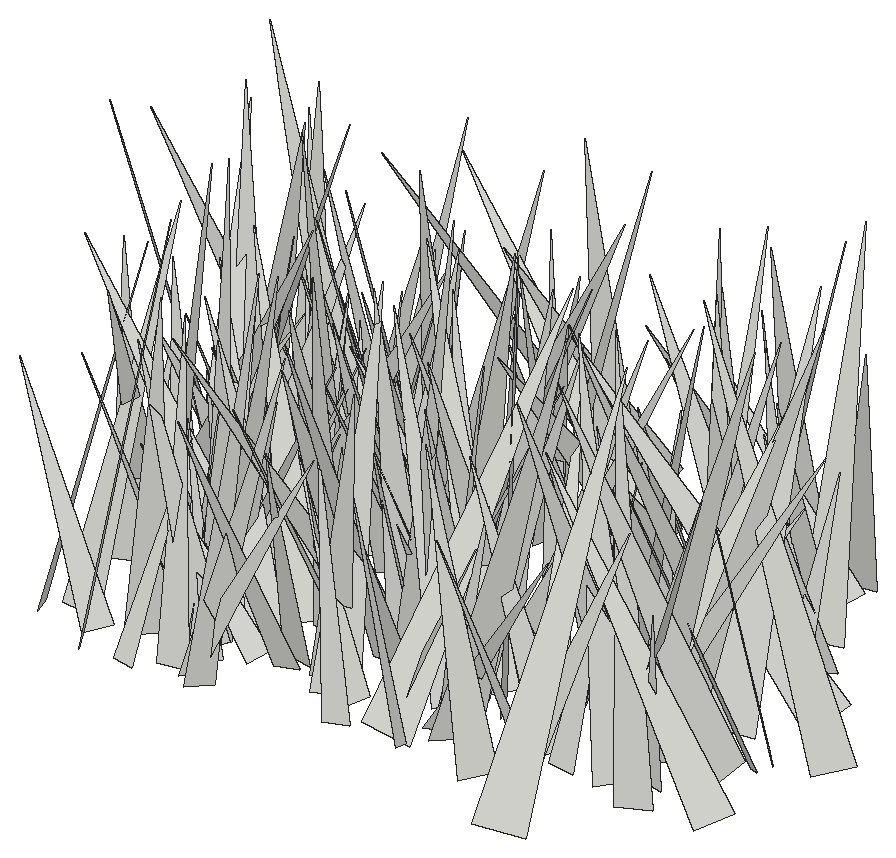
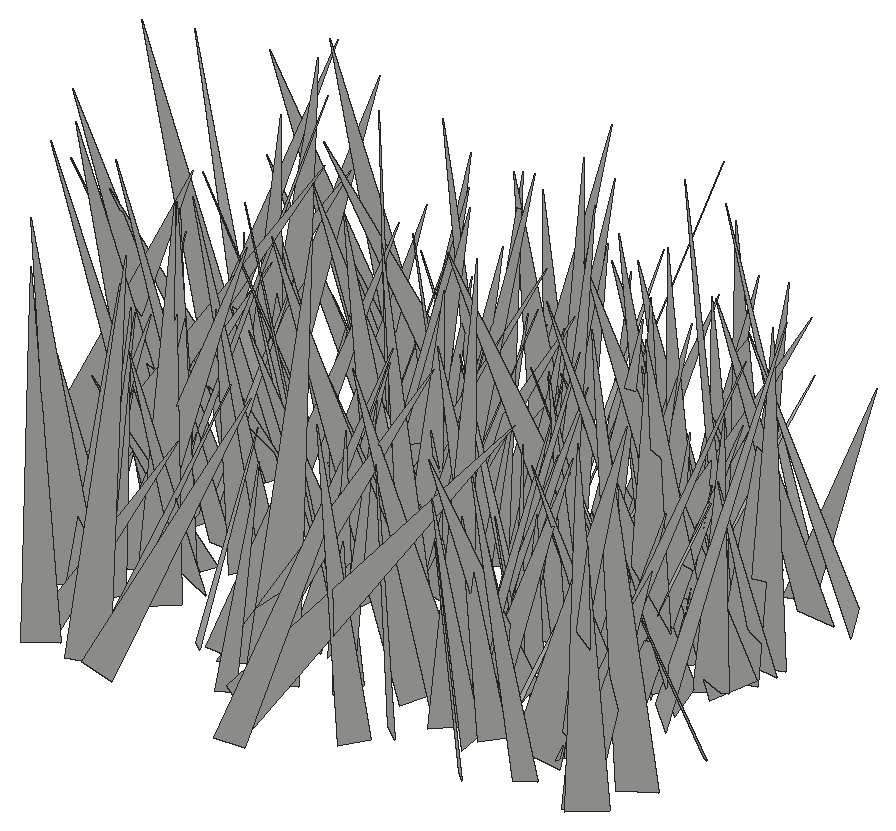
# SketchUp Ruby script. Lengths in inches.
U = 1.inch
M = Sketchup.active_model
def pt(a) = Geom::Point3d.new(a.map { |v| v * U })
def face(e, loops, mat)
  f = e.add_face(loops[0].map { |a| pt(a) })
  loops[1..].each { |l| e.add_face(l.map { |a| pt(a) }).erase! }
  f.material = f.back_material = mat if mat
  f
end
# faces: each face lists its corners as indices into pts; further lists are holes
def faces(e, pts, list, mat = nil) = list.each { |f| face(e, (f[0].is_a?(Array) ? f : [f]).map { |l| l.map { |i| pts[i] } }, mat) }
# xy, xz, yz: faces in a plane at the given z, y or x. An outline is a flat list of corners, or four numbers for a rectangle; further outlines are holes
def ring(l) = l.size == 4 ? [[l[0], l[1]], [l[2], l[1]], [l[2], l[3]], [l[0], l[3]]] : l.each_slice(2).to_a
def flat(e, list, mat, &to3) = list.each { |f| face(e, (f[0].is_a?(Array) ? f : [f]).map { |l| ring(l).map { |u, v| to3.(u, v) } }, mat) }
def xy(e, z, list, mat = nil) = flat(e, list, mat) { |x, y| [x, y, z] }
def xz(e, y, list, mat = nil) = flat(e, list, mat) { |x, z| [x, y, z] }
def yz(e, x, list, mat = nil) = flat(e, list, mat) { |y, z| [x, y, z] }
def lines(e, pts, list) = list.each { |a, b| e.add_line(pt(pts[a]), pt(pts[b])) }
# prism: a flat outline (further loops are holes) pulled along v
def prism(e, loops, v, mat = nil)
  f = face(e, loops, mat); d = Geom::Vector3d.new(v.map { |x| x * U })
  f.pushpull(f.normal.samedirection?(d) ? d.length : -d.length)
end
def box(e, o, s, mat = nil) = prism(e, [[o, [o[0] + s[0], o[1], o[2]], [o[0] + s[0], o[1] + s[1], o[2]], [o[0], o[1] + s[1], o[2]]]], [0, 0, s[2]], mat)
def at(x, y, z, deg = 0) = Geom::Transformation.translation(pt([x, y, z])) * Geom::Transformation.rotation(ORIGIN, Z_AXIS, deg.degrees)
def axes(o, x, y, z) = Geom::Transformation.new([*x, 0, *y, 0, *z, 0, *pt(o).to_a, 1])
def part(name) = M.definitions.add(name)
# library, detail: a bought-in or finely detailed component or shape, given as its bounding box
def library(name, o, s) = part(name).tap { |d| box(d.entities, o, s) }
def detail(e, o, s) = box(e.add_group.entities, o, s)
def put(e, d, t, mat = nil) = e.add_instance(d, t).tap { |i| i.material = mat if mat }
def group(e, t, mat = nil) = e.add_group.tap { |g| g.transformation = t; g.material = mat if mat }.entities
root = M.entities
c1 = part("fur_instance\#9")
p = [[0.8125,0,1.79],[0.67,-0.02,1.48],[0,-0.11,0],[0,0.11,0]]
faces(c1.entities,p,[[0,1,2,3]])
put(root,c1,axes([129.59,252.91,-27.1],[-4.54367,3.48057,1.82928],[3.81076,4.58683,0.73803],[0.96889,-1.71821,5.67579]))
put(root,c1,axes([114.01,252.82,-27.1],[-3.48001,3.233,0.8636],[3.33945,3.27515,1.19585],[-0.21495,-1.45934,4.59703]))
put(root,c1,axes([117.92,252.73,-27.1],[2.74788,4.31889,0.7575],[4.17328,-2.30167,-2.01583],[1.34551,-1.68135,4.70533]))
put(root,c1,axes([116.02,251.58,-27.1],[0.74131,3.87524,0.12897],[3.87698,-0.74271,0.03187],[-0.05555,-0.12068,3.94537]))
put(root,c1,axes([115.4,253.56,-27.1],[-4.12278,4.06528,3.37823],[4.64279,4.83304,-0.14992],[2.52655,-2.24755,5.78803]))
put(root,c1,axes([120.35,254.6,-27.1],[-0.32554,-5.06602,0.7464],[-4.99056,0.14633,-1.18345],[-1.14716,0.80105,4.9366]))
put(root,c1,axes([132.36,250.52,-27.1],[-3.86216,7.0455,1.20437],[6.7899,4.04407,-1.88376],[2.2331,-0.11104,7.81068]))
put(root,c1,axes([123.87,252.73,-27.1],[-0.78367,4.54033,1.31363],[4.69244,0.5877,0.76808],[-0.56674,-1.41222,4.54299]))
put(root,c1,axes([113.97,252.05,-27.1],[6.26441,4.08516,1.86388],[4.05019,-6.52197,0.68206],[-1.9387,-0.42509,7.44756]))
put(root,c1,axes([117.64,254.12,-27.1],[-4.95355,2.49117,1.9463],[2.93301,4.97148,1.10159],[1.17959,-1.90003,5.43416]))
put(root,c1,axes([130.23,254.6,-27.1],[-3.91317,-2.34388,0.53173],[-2.28614,3.94348,0.55853],[0.74167,-0.21123,4.52711]))
put(root,c1,axes([117.44,252.4,-27.1],[-0.20928,5.81187,1.2771],[5.90875,0.05179,0.73257],[-0.70395,-1.2931,5.76932]))
put(root,c1,axes([118.37,252.4,-27.1],[5.34451,-1.51745,2.02584],[-2.07356,-5.33917,1.4711],[-1.45157,2.03988,5.35746]))
put(root,c1,axes([131.07,252.87,-27.1],[0.51844,5.23573,1.343],[5.13497,-0.0558,-1.76472],[1.68777,-1.43851,4.95655]))
put(root,c1,axes([120.26,255.23,-27.1],[0.02895,-4.95019,0.58964],[-4.94989,0.0415,0.59139],[0.59214,0.58889,4.91483]))
put(root,c1,axes([126.4,252.91,-27.1],[-4.21104,-1.2398,0.43934],[-1.31531,3.95873,-1.43574],[-0.00925,1.50143,4.14832]))
put(root,c1,axes([125.05,254.18,-27.1],[3.85978,2.30102,0.3483],[2.28006,-3.60384,-1.45862],[0.46617,-1.42533,4.2503]))
put(root,c1,axes([117.06,254.07,-27.1],[-4.69197,-2.31538,0.05263],[-2.28134,4.60011,-1.00642],[-0.39908,0.92541,5.13447]))
put(root,c1,axes([121.87,254.95,-27.1],[3.13383,-5.16211,1.39491],[-5.34355,-3.08346,0.59403],[-0.19921,1.50298,6.00961]))
put(root,c1,axes([118.89,251.94,-27.1],[-6.51752,1.2418,2.00991],[0.54856,6.53189,-2.25684],[2.29801,1.9627,6.23913]))
put(root,c1,axes([119.2,254.6,-27.1],[-3.24563,2.42896,0.17461],[2.25293,2.88449,1.75171],[-0.92447,-1.49811,3.65588]))
put(root,c1,axes([122.88,256.92,-27.1],[-0.43608,-7.58063,0.50958],[-7.59761,0.43802,0.01424],[0.04352,0.50791,7.59315]))
put(root,c1,axes([118.24,253.43,-27.1],[-3.93894,0.78438,0.2139],[0.7314,3.88076,-0.76228],[0.35506,0.70765,3.94328]))
put(root,c1,axes([123.49,254.3,-27.1],[-4.0044,1.49429,0.5536],[1.5481,4.00291,0.3933],[0.37782,-0.56428,4.25599]))
put(root,c1,axes([122.49,255.03,-27.1],[-1.30736,-3.53096,1.01989],[-3.67333,1.2908,-0.2398],[0.12042,1.04076,3.75757]))
put(root,c1,axes([121.07,256.91,-27.1],[-3.83453,-4.44323,0.31037],[-4.29048,3.7947,1.3169],[1.19597,-0.63261,5.71941]))
put(root,c1,axes([126.65,254.46,-27.1],[3.7348,-2.45498,0.02516],[-2.33086,-3.53122,1.44009],[0.77113,1.21649,4.23106]))
put(root,c1,axes([117.09,253.32,-27.1],[2.12896,3.50938,0.78952],[3.35263,-2.26833,1.04217],[-1.30344,-0.10245,3.97015]))
put(root,c1,axes([127.47,254.32,-27.1],[7.2049,-3.47591,1.96261],[-3.83046,-7.15988,1.38131],[-1.1231,2.12096,7.87937]))
put(root,c1,axes([119.89,259.11,-27.1],[-6.50454,-4.83681,0.42708],[-4.2184,5.98256,3.50717],[2.40464,-2.5885,7.30777]))
put(root,c1,axes([111.64,252.9,-27.1],[5.51365,3.20537,1.24598],[2.89904,-5.59864,1.57419],[-1.84998,0.77981,6.18035]))
put(root,c1,axes([130.52,255.7,-27.1],[-4.35819,2.96505,1.59627],[3.3258,4.19926,1.28011],[0.52792,-1.97688,5.11338]))
put(root,c1,axes([133.25,257,-27.1],[1.43067,-7.01564,1.7352],[-6.90944,-1.84641,-1.76845],[-2.11892,1.28394,6.9382]))
put(root,c1,axes([137.39,255.32,-27.1],[-4.14935,5.21761,0.66717],[4.85978,3.47746,3.02911],[-2.01273,-2.35998,5.93844]))
put(root,c1,axes([120.62,258.33,-27.1],[5.40488,-4.57462,0.50738],[-4.27322,-5.27816,-2.06831],[-1.71004,-1.26929,6.77215]))
put(root,c1,axes([122.66,254.21,-27.1],[-3.77046,5.93467,2.17976],[6.06315,4.1134,-0.71146],[1.79161,-1.43096,6.99504]))
put(root,c1,axes([134.34,255.89,-27.1],[-0.14412,-3.47359,1.04669],[-3.58722,0.2928,0.47779],[0.54152,1.01518,3.44359]))
put(root,c1,axes([132.18,257.37,-27.1],[7.41722,0.99885,0.34739],[1.05742,-6.96886,-2.53978],[0.01548,-2.56338,7.04006]))
put(root,c1,axes([126.39,255.35,-27.1],[0.00091,-3.67707,1.93886],[-4.08733,0.35251,0.67045],[0.75747,1.90654,3.61543]))
put(root,c1,axes([112.81,253.43,-27.1],[0.72086,7.11073,0.81641],[7.15729,-0.71063,-0.13028],[0.04812,-0.82534,7.14599]))
put(root,c1,axes([133.4,255.4,-27.1],[-5.88987,4.84378,2.23578],[5.14185,6.04195,0.45575],[1.42207,-1.78441,7.61217]))
put(root,c1,axes([131.36,254.9375,-27.1],[0.22863,4.55848,1.01522],[4.65358,-0.13679,-0.43379],[0.39321,-1.03161,4.54355]))
put(root,c1,axes([135.82,257.82,-27.1],[-7.8024,0.71377,1.7229],[1.19599,7.6017,2.26696],[1.43089,-2.46171,7.49986]))
put(root,c1,axes([112.16,258.375,-27.1],[2.77965,-6.05851,0.20454],[-6.05263,-2.78627,-0.276],[-0.3362,0.0706,6.66001]))
put(root,c1,axes([118,256.51,-27.1],[-6.653,2.83628,0.09553],[2.75112,6.38619,1.99099],[-0.69638,-1.86767,6.95291]))
put(root,c1,axes([120.18,257.19,-27.1],[-0.4517,-7.27096,2.0225],[-7.50286,0.65147,0.6664],[0.81515,1.96726,7.25444]))
put(root,c1,axes([116.52,256.22,-27.1],[6.38697,-1.69717,1.73981],[-1.81592,-6.58358,0.24416],[-1.61547,0.69051,6.6041]))
put(root,c1,axes([125.53,253.21,-27.1],[-1.37451,8.097,0.63904],[7.82187,1.49419,-2.10823],[2.18815,-0.25501,7.93763]))
put(root,c1,axes([126.71,254.72,-27.1],[3.29752,4.92899,1.52703],[4.76096,-3.60504,1.35547],[-1.98997,-0.45731,5.77332]))
put(root,c1,axes([113.85,256.53,-27.1],[4.80804,6.17674,2.98381],[6.78482,-4.81897,-0.95722],[-1.01068,-2.96612,7.76873]))
put(root,c1,axes([134.84,254.35,-27.1],[-0.02832,7.80203,1.3013],[7.5934,-0.33756,2.1891],[-2.2148,-1.25708,7.48868]))
put(root,c1,axes([117.64,254.31,-27.1],[-7.86516,0.65945,1.92725],[0.13584,7.83978,-2.12819],[2.03241,2.02799,7.60042]))
put(root,c1,axes([116.55,256.39,-27.1],[3.89931,-1.45547,0.98195],[-1.58431,-3.9476,0.44006],[-0.75669,0.76505,4.13877]))
put(root,c1,axes([112.03,257.02,-27.1],[2.29625,-5.32789,2.30917],[-5.72704,-2.48806,-0.04565],[-0.95905,2.10109,5.80148]))
put(root,c1,axes([123.34,257.37,-27.1],[3.99451,-5.40043,2.70776],[-5.64329,-4.49426,-0.63847],[-2.15638,1.75774,6.68679]))
put(root,c1,axes([123.23,257.58,-27.1],[-1.72033,-4.15588,1.09836],[-4.2769,1.77348,0.01157],[0.4311,1.01028,4.49785]))
put(root,c1,axes([116.7,256.26,-27.1],[0.17252,3.92598,1.26935],[3.97591,-0.49782,0.99933],[-1.10305,-1.18034,3.80058]))
put(root,c1,axes([125.57,257.53,-27.1],[-2.41735,-5.08882,0.8159],[-4.81582,1.90935,-2.35956],[-1.83565,1.69223,5.11586]))
put(root,c1,axes([117.93,257.56,-27.1],[-5.02237,2.51021,1.68016],[2.86774,4.98644,1.12241],[0.94877,-1.78398,5.50142]))
put(root,c1,axes([125.96,256.1,-27.1],[-6.07575,2.79462,0.62219],[2.80321,6.10345,-0.04049],[0.58225,-0.22305,6.68752]))
put(root,c1,axes([123.87,256.27,-27.1],[3.41828,7.22194,2.57308],[7.56489,-3.63472,0.1519],[-1.24484,-2.25703,7.98861]))
put(root,c1,axes([115.95,256.41,-27.1],[-2.49427,4.27012,1.59064],[4.35584,2.76683,-0.59729],[1.33819,-1.04698,4.90903]))
put(root,c1,axes([118.85,255.46,-27.1],[-2.09774,5.99421,0.07606],[5.73274,1.98235,1.88224],[-1.75272,-0.69034,6.06533]))
put(root,c1,axes([116.13,256.1,-27.1],[4.9565,-0.0282,0.53243],[-0.1703,-4.80111,1.33099],[-0.50525,1.34155,4.77453]))
put(root,c1,axes([124.52,258.66,-27.1],[-3.87512,-3.17972,0.32504],[-3.163,3.88842,0.32938],[0.4601,-0.04943,5.00187]))
put(root,c1,axes([121.32,259.05,-27.1],[-2.38013,-2.88459,0.25848],[-2.75196,2.35686,0.96161],[0.90246,-0.42079,3.61403]))
put(root,c1,axes([125.82,259.48,-27.1],[3.87648,-5.20572,1.47803],[-5.00062,-4.14086,-1.46909],[-2.0683,0.2548,6.32205]))
put(root,c1,axes([127.39,256.97,-27.1],[6.18055,4.14964,3.19418],[4.26505,-6.85588,0.65402],[-3.03836,-1.18276,7.41558]))
put(root,c1,axes([125.02,258.51,-27.1],[-0.19276,-5.01478,1.27598],[-5.16585,0.1124,-0.33865],[-0.30027,1.28555,5.00705]))
put(root,c1,axes([118.4,259.92,-27.1],[4.15376,-5.21591,0.7578],[-5.12927,-4.22232,-0.94677],[-1.21268,-0.00681,6.60024]))
put(root,c1,axes([126.24,256.61,-27.1],[6.10707,-2.19869,2.10682],[-2.76305,-5.98564,1.76265],[-1.28003,2.43046,6.24689]))
put(root,c1,axes([123.23,260.01,-27.1],[-2.01035,-7.12989,1.00319],[-7.18316,2.0575,0.22838],[0.49393,0.90254,7.40437]))
put(root,c1,axes([132.33,257.89,-27.1],[6.94828,-4.27135,1.74082],[-4.55894,-6.83788,1.41876],[-0.70067,2.13364,8.03182]))
put(root,c1,axes([126.39,259.63,-27.1],[-6.42762,0.7775,0.36666],[0.8533,6.10569,2.01137],[0.10407,-2.04186,6.15412]))
put(root,c1,axes([118.98,257.37,-27.1],[-4.49285,4.90641,0.97236],[5.00159,4.41981,0.80831],[0.04935,-1.26349,6.60342]))
put(root,c1,axes([111.85,257.19,-27.1],[0.3484,4.1984,0.59349],[4.23915,-0.35779,0.04247],[-0.09183,-0.58788,4.21262]))
put(root,c1,axes([126.6,257.47,-27.1],[-5.45873,5.352,1.02249],[5.44819,5.38274,0.9113],[0.08123,-1.36725,7.5902]))
put(root,c1,axes([136.29,258.72,-27.1],[-3.48224,-3.77241,0.29956],[-3.58403,3.15695,-1.90663],[-1.21472,1.49981,4.76674]))
put(root,c1,axes([116.47,258.5625,-27.1],[3.59656,-0.31618,0.04156],[-0.31764,-3.59357,0.14939],[-0.02828,0.15246,3.60734]))
put(root,c1,axes([118.32,259.29,-27.1],[-3.2308,-2.41105,0.08917],[-2.40238,3.20101,-0.49122],[-0.22293,0.4467,4.00124]))
put(root,c1,axes([114.16,259.76,-27.1],[3.91302,0.34843,0.25725],[0.41449,-3.69091,-1.30566],[-0.12562,-1.32482,3.70519]))
put(root,c1,axes([111.92,258.78,-27.1],[6.68383,-3.60485,0.36068],[-3.59385,-6.50181,1.61538],[0.45749,1.59067,7.42019]))
put(root,c1,axes([130.04,258.8,-27.1],[-4.57594,-0.69447,0.70937],[-0.73517,4.61906,-0.2203],[0.6671,0.32667,4.62309]))
put(root,c1,axes([115.96,258.54,-27.1],[4.04604,3.23344,0.3968],[3.2461,-3.94826,-0.92578],[0.27467,-0.96906,5.09593]))
put(root,c1,axes([115.92,260.46,-27.1],[0.4513,-4.46287,0.47479],[-4.46772,-0.49211,-0.3789],[-0.42669,0.43236,4.4696]))
put(root,c1,axes([132.03,260.8,-27.1],[-2.1706,-3.79382,0.07549],[-3.76138,2.16267,0.53397],[0.50075,-0.20018,4.33814]))
put(root,c1,axes([113.86,259.62,-27.1],[2.36967,1.89121,2.13493],[2.35412,-2.86396,-0.07595],[-1.61018,-1.40392,3.03088]))
put(root,c1,axes([124.71,257.41,-27.1],[0.6459,3.9486,0.07217],[3.68247,-0.62859,1.43463],[-1.42692,0.16515,3.73504]))
put(root,c1,axes([136.28,259.63,-27.1],[-3.38614,-3.10021,1.02366],[-3.22386,3.40798,-0.34286],[0.51569,0.94841,4.57818]))
put(root,c1,axes([112.42,259.33,-27.1],[2.60909,-3.89298,2.22887],[-4.24925,-2.97119,-0.21539],[-1.4377,1.71676,4.68148]))
put(root,c1,axes([132.41,256.97,-27.1],[-1.13308,6.40977,0.66119],[6.08836,1.28481,-2.02171],[2.11049,-0.26515,6.18722]))
put(root,c1,axes([113.86,261.7,-27.1],[3.91388,-2.85851,1.41513],[-2.09693,-3.9939,-2.26798],[-2.40345,-1.17037,4.2832]))
put(root,c1,axes([118.05,258.32,-27.1],[0.83118,5.18677,1.07004],[5.28228,-0.88982,0.21009],[-0.38088,-1.02179,5.24874]))
put(root,c1,axes([129.16,259.1,-27.1],[-3.23487,-1.73884,2.61208],[-2.22596,3.91581,-0.14997],[2.2117,1.39779,3.66954]))
put(root,c1,axes([118.47,259.98,-27.1],[-2.90002,-7.26429,3.03178],[-7.85451,2.88308,-0.60516],[0.51793,3.0479,7.79832]))
put(root,c1,axes([115.9375,259.31,-27.1],[5.9864,-4.39629,0.74457],[-4.35138,-5.48795,2.58196],[0.97326,2.50473,6.96403]))
put(root,c1,axes([132.49,262.61,-27.1],[-7.22673,-3.69522,1.05519],[-3.3656,7.17065,2.06111],[1.85494,-1.38592,7.85061]))
put(root,c1,axes([122.51,259.36,-27.1],[4.96423,2.67259,0.04648],[2.6631,-4.93667,-0.5706],[0.22978,-0.52435,5.60898]))
put(root,c1,axes([131.36,259.56,-27.1],[4.19059,5.13354,0.34706],[4.85008,-3.79176,-2.47669],[1.71767,-1.81771,6.14657]))
put(root,c1,axes([119.16,261.63,-27.1],[1.67149,-5.33301,0.8085],[-5.34441,-1.75188,-0.5067],[-0.72935,0.6152,5.5658]))
put(root,c1,axes([115.84,260.74,-27.1],[-3.47734,-1.80435,0.22841],[-1.8088,3.48242,-0.02761],[0.19,0.12974,3.9175]))
put(root,c1,axes([124.07,259.72,-27.1],[-4.47005,3.93119,1.60818],[4.11701,4.5843,0.23722],[1.04438,-1.24571,5.94805]))
put(root,c1,axes([112.61,261.66,-27.1],[-5.20648,-5.71637,1.32602],[-5.85189,5.18966,-0.6046],[0.43665,1.3904,7.70836]))
put(root,c1,axes([114.8,261.06,-27.1],[-3.58425,-2.16039,0.18109],[-2.16614,3.55434,-0.47063],[-0.08907,0.49634,4.15845]))
put(root,c1,axes([114.11,258.43,-27.1],[-5.29033,5.65073,1.03717],[5.57546,5.38985,-0.92613],[1.38587,-0.11308,7.68509]))
put(root,c1,axes([136.13,262.8,-27.1],[-7.44265,2.94787,0.75024],[2.95668,6.54484,3.6151],[-0.71474,-3.62229,7.14241]))
put(root,c1,axes([124.03,260.9,-27.1],[5.12868,-4.19399,1.94705],[-4.5125,-5.17419,0.74098],[-1.00889,1.82269,6.58361]))
put(root,c1,axes([125.23,260.5,-27.1],[5.08074,5.57509,0.64514],[5.46993,-4.72427,-2.25231],[1.25607,-1.97773,7.19879]))
put(root,c1,axes([115.9,261.69,-27.1],[-0.80392,-5.00028,1.94874],[-5.12712,1.2977,1.21465],[1.58527,1.66129,4.91668]))
put(root,c1,axes([131.92,260.36,-27.1],[6.06814,-4.77445,2.10475],[-5.2154,-5.64781,2.22478],[-0.15808,3.05854,7.39379]))
put(root,c1,axes([114.03,260.28,-27.1],[4.42151,2.80893,1.55928],[2.73673,-4.68252,0.67492],[-1.68278,-0.23477,5.19464]))
put(root,c1,axes([127.21,259.64,-27.1],[-2.44616,4.11048,0.29857],[4.09909,2.46258,-0.31948],[0.42742,-0.0923,4.7726]))
put(root,c1,axes([138.32,260.3,-27.1],[-2.68904,7.46116,1.26428],[7.06219,1.99214,3.26422],[-2.71897,-2.20471,7.22805]))
put(root,c1,axes([113.89,260.73,-27.1],[5.91163,-3.56463,4.13587],[-4.286,-6.80601,0.26026],[-3.38262,2.39395,6.89828]))
put(root,c1,axes([122.27,263.15,-27.1],[-5.24413,-0.63684,1.6828],[-0.10679,5.28634,1.66778],[1.7961,-1.54509,5.01248]))
put(root,c1,axes([129.49,260.9375,-27.1],[6.35559,1.23086,1.81432],[1.1106,-6.60444,0.5901],[-1.89033,0.25813,6.44673]))
put(root,c1,axes([112.67,260.33,-27.1],[7.43833,2.19546,1.23858],[2.06036,-7.51855,0.95355],[-1.45225,0.57818,7.69672]))
put(root,c1,axes([119.25,262.4,-27.1],[-2.70694,-4.99144,1.16007],[-5.08628,2.45713,-1.29614],[-0.62448,1.62351,5.52829]))
put(root,c1,axes([117.57,262.19,-27.1],[5.27684,1.71083,0.85913],[1.8324,-5.24307,-0.81398],[-0.55438,-1.04563,5.4872]))
put(root,c1,axes([134.07,260.2,-27.1],[-2.77927,7.20298,1.80131],[7.21654,3.07297,-1.15349],[1.74623,-1.2353,7.63392]))
put(root,c1,axes([118.89,262.9375,-27.1],[-4.07714,-4.72232,1.18622],[-4.85623,4.056,-0.54439],[0.3528,1.25658,6.21506]))
put(root,c1,axes([130.67,261.6875,-27.1],[2.74298,6.25055,1.8619],[6.47418,-2.36552,-1.59662],[0.78801,-2.32269,6.63657]))
put(root,c1,axes([117.35,263.09,-27.1],[-1.65671,-3.63214,1.3485],[-3.6613,1.94738,0.7471],[1.26719,0.87797,3.92161]))
put(root,c1,axes([129.11,262.48,-27.1],[-3.54773,2.23846,2.32232],[2.39169,4.14191,-0.33862],[2.16418,-0.90784,4.1812]))
put(root,c1,axes([126.16,267.15,-27.1],[6.60243,-3.6292,1.16999],[-2.40466,-5.77841,-4.35427],[-2.95933,-3.40161,6.14845]))
put(root,c1,axes([119.12,262.07,-27.1],[3.9195,-3.82723,2.46639],[-4.43668,-3.94163,0.93419],[-1.02305,2.43088,5.39791]))
put(root,c1,axes([120.66,263.87,-27.1],[0.32033,-6.88611,1.90206],[-6.92731,0.16595,1.76741],[1.74605,1.92169,6.66313]))
put(root,c1,axes([109.84,262.84,-27.1],[3.27011,3.05252,0.13659],[2.8317,-2.95233,-1.81533],[1.14804,-1.41282,4.08853]))
put(root,c1,axes([117.72,261.96,-27.1],[-2.46678,3.0111,0.36551],[3.02886,2.4705,0.08915],[0.1623,-0.33942,3.8915]))
put(root,c1,axes([118.68,263.64,-27.1],[-2.89225,-3.68575,0.79235],[-3.76683,2.78458,-0.79678],[-0.15371,1.11313,4.61682]))
put(root,c1,axes([113.37,265.42,-27.1],[-7.55604,-1.18176,1.01335],[-0.88861,7.39753,2.00103],[1.27821,-1.84315,7.38147]))
put(root,c1,axes([124.77,262.24,-27.1],[4.76351,-2.22786,1.63166],[-2.67424,-4.53288,1.61806],[-0.68857,2.19233,5.00362]))
put(root,c1,axes([132.32,261.52,-27.1],[-7.61718,0.0241,1.98426],[-0.51537,7.57673,-2.07045],[1.91631,2.1335,7.33043]))
put(root,c1,axes([121.25,262.55,-27.1],[6.06997,0.80019,0.53139],[0.73411,-6.05703,0.73529],[-0.61948,0.66277,6.07817]))
put(root,c1,axes([127.07,264.11,-27.1],[1.11597,-3.30458,1.27259],[-3.40234,-1.37051,-0.57526],[-0.98175,0.99326,3.44016]))
put(root,c1,axes([130.07,263.08,-27.1],[0.48143,3.7055,0.846],[3.27794,0.02687,-1.98307],[1.92393,-0.97302,3.16701]))
put(root,c1,axes([124.44,265.1,-27.1],[0.3349,-5.08877,0.86463],[-5.08924,-0.4702,-0.79617],[-0.86188,0.79915,5.03725]))
put(root,c1,axes([132.91,261.77,-27.1],[7.20277,3.49638,1.97973],[3.12762,-7.42996,1.74287],[-2.5223,0.77133,7.81454]))
put(root,c1,axes([130.77,264.02,-27.1],[4.6761,-4.10232,2.76945],[-4.45315,-5.14998,-0.1096],[-2.16064,1.73593,6.21956]))
put(root,c1,axes([117.37,262.71,-27.1],[1.88548,3.67223,0.79609],[3.49899,-2.04056,1.12569],[-1.36969,-0.15771,3.97154]))
put(root,c1,axes([117.53,266.34,-27.1],[7.0973,-2.99001,1.53723],[-2.6894,-7.20395,-1.59536],[-2.01752,-0.91535,7.53436]))
put(root,c1,axes([132.13,264.72,-27.1],[-5.92654,3.46188,1.28835],[3.68281,5.72588,1.55549],[0.28525,-1.99951,6.68498]))
put(root,c1,axes([134.06,265.17,-27.1],[0.22156,-4.52657,1.23949],[-4.53883,-0.5223,-1.09609],[-1.19379,1.1457,4.39744]))
put(root,c1,axes([110.2,265.87,-27.1],[1.15039,-7.47242,1.55869],[-7.41634,-0.72104,2.01691],[1.80677,1.79806,7.28646]))
put(root,c1,axes([116.54,264.31,-27.1],[-4.07706,-2.14403,0.24298],[-2.12817,3.90987,-1.20919],[-0.35608,1.18084,4.44491]))
put(root,c1,axes([112.15,263.64,-27.1],[0.82135,5.31818,1.14764],[5.3338,-0.55827,-1.23031],[1.07271,-1.29616,5.2387]))
put(root,c1,axes([111.73,266.77,-27.1],[1.96703,-4.29578,0.10046],[-4.18734,-1.94112,-1.01553],[-0.96439,-0.33368,4.61429]))
put(root,c1,axes([119.4,265.27,-27.1],[5.85705,-5.48153,0.51052],[-5.36351,-5.5136,2.33363],[1.24121,2.04104,7.67505]))
put(root,c1,axes([133.44,264.39,-27.1],[-1.54021,3.23682,1.39983],[3.28512,1.87235,-0.71486],[1.28237,-0.90889,3.51258]))
put(root,c1,axes([129.85,265.97,-27.1],[-4.92901,3.2655,3.81824],[4.17297,5.6397,0.56365],[2.798,-2.65855,5.88565]))
put(root,c1,axes([117.55,264.375,-27.1],[-2.16703,-5.16397,2.37315],[-5.48971,1.24499,-2.30381],[-1.47021,2.96275,5.10441]))
put(root,c1,axes([112.35,265.67,-27.1],[2.0816,-3.74764,1.04429],[-3.88491,-2.06538,0.3318],[-0.20701,1.076,4.27408]))
put(root,c1,axes([117.31,265.76,-27.1],[2.82941,3.82153,3.56935],[4.50896,-3.83832,0.53527],[-2.64833,-2.45217,4.72474]))
put(root,c1,axes([121.68,266.39,-27.1],[4.68677,-2.0034,0.66372],[-1.95488,-4.73014,-0.47351],[-0.79535,-0.17932,5.07496]))
put(root,c1,axes([133.05,265.66,-27.1],[0.28684,-3.45624,1.82339],[-3.70035,-0.82791,-0.9872],[-1.25608,1.64973,3.32465]))
put(root,c1,axes([121.99,266.02,-27.1],[6.05057,5.41917,1.99571],[5.77348,-5.74186,-1.9125],[-0.1309,-2.76104,7.89425]))
put(root,c1,axes([131.96,267.42,-27.1],[4.64418,-2.47093,1.08294],[-2.19439,-4.71399,-1.3452],[-1.56935,-0.72073,5.0857]))
put(root,c1,axes([127.18,267.28,-27.1],[-2.4025,-2.92839,0.44923],[-2.80853,2.4353,0.85486],[0.94311,-0.20767,3.69008]))
put(root,c1,axes([123.61,264.38,-27.1],[-5.70107,0.73605,0.76728],[0.48907,5.53142,-1.67238],[0.94409,1.57933,5.49974]))
put(root,c1,axes([121.36,267.11,-27.1],[-1.65824,-4.82946,1.36253],[-4.95542,1.80194,0.35604],[0.78993,1.16588,5.09379]))
put(root,c1,axes([131.42,266.55,-27.1],[-4.23654,2.45749,2.21286],[2.8358,4.54981,0.37637],[1.70124,-1.46429,4.88322]))
put(root,c1,axes([118.69,265.02,-27.1],[6.30569,-0.68619,2.05979],[-1.17683,-6.39727,1.4715],[-1.82446,1.75482,6.16987]))
put(root,c1,axes([121.23,267,-27.1],[-1.26744,-3.38882,1.28492],[-3.35573,1.6115,0.94004],[1.36901,0.81271,3.49382]))
put(root,c1,axes([130.38,267.52,-27.1],[-4.86082,-0.82699,0.28427],[-0.77768,4.82218,0.73078],[0.39992,-0.67448,4.87621]))
put(root,c1,axes([116.79,263.49,-27.1],[-6.46453,1.71895,1.7422],[0.79023,6.12289,-3.109],[2.31637,2.70842,5.92275]))
put(root,c1,axes([131.86,266.375,-27.1],[-3.13424,-4.33981,2.11732],[-4.81159,3.01955,-0.93345],[0.40688,2.2779,5.27125]))
put(root,c1,axes([115.95,266.13,-27.1],[2.7326,-2.75522,2.01665],[-3.2693,-2.85632,0.52755],[-0.98478,1.83723,3.84448]))
put(root,c1,axes([123.83,267.66,-27.1],[3.74176,-6.61768,2.63887],[-6.89022,-4.11933,-0.5604],[-1.81167,1.99888,7.58159]))
put(root,c1,axes([114.12,266.2,-27.1],[-2.60972,7.0339,1.93347],[7.14895,2.0575,2.16424],[-1.45142,-2.51309,7.18348]))
put(root,c1,axes([125.45,267.27,-27.1],[-6.72983,3.60579,0.05795],[3.45053,6.40273,2.3226],[-1.04828,-2.07339,7.27309]))
put(root,c1,axes([111.04,268.04,-27.1],[2.15592,-3.18911,0.31319],[-3.19535,-2.16794,-0.07942],[-0.24138,0.21478,3.84865]))
put(root,c1,axes([113.45,267.6,-27.1],[0.14432,-5.01914,1.5992],[-4.96199,0.40759,1.72702],[1.76858,1.55311,4.71487]))
put(root,c1,axes([130.01,264.09,-27.1],[1.21236,6.8418,0.01969],[6.58716,-1.17263,1.87473],[-1.84929,0.30844,6.6907]))
put(root,c1,axes([116.36,266.72,-27.1],[4.45017,0.43948,1.54669],[0.28501,-4.6951,0.51402],[-1.58245,0.39027,4.44218]))
put(root,c1,axes([112.84,265.72,-27.1],[-0.8171,5.77252,0.59098],[5.63961,0.64951,1.4532],[-1.36602,-0.77139,5.64605]))
put(root,c1,axes([124.64,269.02,-27.1],[3.47774,-1.50181,0.39234],[-1.2719,-3.30895,-1.39185],[-0.88975,-1.13996,3.5232]))
put(root,c1,axes([110.64,267.89,-27.1],[3.75494,-4.9741,2.2471],[-5.32599,-3.93562,0.18806],[-1.1937,1.91308,6.22943]))
put(root,c1,axes([118.77,267.83,-27.1],[2.85129,3.39796,1.84964],[3.79237,-2.9092,-0.50161],[-0.76499,-1.75715,4.40731]))
put(root,c1,axes([132.7,266.61,-27.1],[-2.30774,6.81626,2.09214],[7.04491,2.51871,-0.43516],[1.09893,-1.8327,7.18315]))
put(root,c1,axes([123.64,269.5,-27.1],[-2.19661,-7.3796,0.4517],[-6.30745,1.62463,-4.13089],[-3.85727,1.54587,6.49764]))
put(root,c1,axes([122.45,271.5625,-27.1],[6.08199,-2.63161,2.26399],[-1.13407,-5.82276,-3.72169],[-3.281,-2.8656,5.48316]))
put(root,c1,axes([119.32,269.05,-27.1],[4.77577,-2.2799,0.31782],[-2.26651,-4.78515,-0.26858],[-0.40236,-0.10607,5.28524]))
put(root,c1,axes([115.26,268.66,-27.1],[2.93725,2.51058,1.33666],[2.80043,-2.8887,-0.72813],[-0.49727,-1.43859,3.79478]))
put(root,c1,axes([131.31,270.22,-27.1],[2.32461,-5.72045,0.33614],[-5.68592,-2.25756,0.90225],[0.71192,0.64824,6.10846]))
put(root,c1,axes([128.68,270.59,-27.1],[0.56796,-5.36738,0.34113],[-5.01782,-0.65229,-1.90884],[-1.93561,0.11605,5.04853]))
put(root,c1,axes([131.78,269.35,-27.1],[-4.01783,2.35497,0.3103],[2.27352,3.63609,1.84258],[-0.68795,-1.73727,4.27712]))
put(root,c1,axes([129.34,270.27,-27.1],[2.40943,-6.40182,1.38295],[-6.51779,-2.4885,-0.16399],[-0.64358,1.23501,6.83826]))
